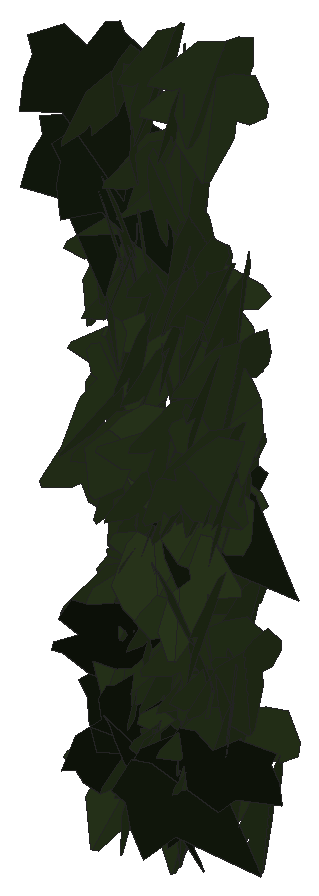
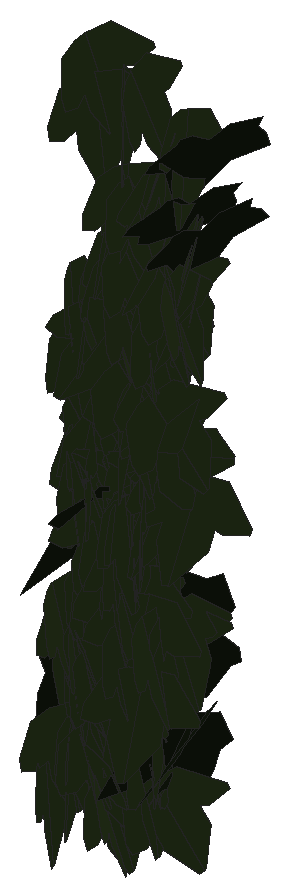
# SketchUp Ruby script. Lengths in inches.
U = 1.inch
M = Sketchup.active_model
def pt(a) = Geom::Point3d.new(a.map { |v| v * U })
def face(e, loops, mat)
  f = e.add_face(loops[0].map { |a| pt(a) })
  loops[1..].each { |l| e.add_face(l.map { |a| pt(a) }).erase! }
  f.material = f.back_material = mat if mat
  f
end
# faces: each face lists its corners as indices into pts; further lists are holes
def faces(e, pts, list, mat = nil) = list.each { |f| face(e, (f[0].is_a?(Array) ? f : [f]).map { |l| l.map { |i| pts[i] } }, mat) }
# xy, xz, yz: faces in a plane at the given z, y or x. An outline is a flat list of corners, or four numbers for a rectangle; further outlines are holes
def ring(l) = l.size == 4 ? [[l[0], l[1]], [l[2], l[1]], [l[2], l[3]], [l[0], l[3]]] : l.each_slice(2).to_a
def flat(e, list, mat, &to3) = list.each { |f| face(e, (f[0].is_a?(Array) ? f : [f]).map { |l| ring(l).map { |u, v| to3.(u, v) } }, mat) }
def xy(e, z, list, mat = nil) = flat(e, list, mat) { |x, y| [x, y, z] }
def xz(e, y, list, mat = nil) = flat(e, list, mat) { |x, z| [x, y, z] }
def yz(e, x, list, mat = nil) = flat(e, list, mat) { |y, z| [x, y, z] }
def lines(e, pts, list) = list.each { |a, b| e.add_line(pt(pts[a]), pt(pts[b])) }
# prism: a flat outline (further loops are holes) pulled along v
def prism(e, loops, v, mat = nil)
  f = face(e, loops, mat); d = Geom::Vector3d.new(v.map { |x| x * U })
  f.pushpull(f.normal.samedirection?(d) ? d.length : -d.length)
end
def box(e, o, s, mat = nil) = prism(e, [[o, [o[0] + s[0], o[1], o[2]], [o[0] + s[0], o[1] + s[1], o[2]], [o[0], o[1] + s[1], o[2]]]], [0, 0, s[2]], mat)
def at(x, y, z, deg = 0) = Geom::Transformation.translation(pt([x, y, z])) * Geom::Transformation.rotation(ORIGIN, Z_AXIS, deg.degrees)
def axes(o, x, y, z) = Geom::Transformation.new([*x, 0, *y, 0, *z, 0, *pt(o).to_a, 1])
def part(name) = M.definitions.add(name)
# library, detail: a bought-in or finely detailed component or shape, given as its bounding box
def library(name, o, s) = part(name).tap { |d| box(d.entities, o, s) }
def detail(e, o, s) = box(e.add_group.entities, o, s)
def put(e, d, t, mat = nil) = e.add_instance(d, t).tap { |i| i.material = mat if mat }
def group(e, t, mat = nil) = e.add_group.tap { |g| g.transformation = t; g.material = mat if mat }.entities
root = M.entities
M.materials.add("efeu1").color = [18, 25, 13]
M.materials.add("efeu2").color = [43, 57, 29]
c1 = part("ivyleaf_10")
p = [[0,0.5,-0.03],[-0.0625,2.02,-0.43],[-0.19,2.01,-0.46],[-0.54,1.05,-0.29],[-0.52,0.625,-0.18],[-0.83,0.76,-0.28],
  [-1.16,0.64,-0.33],[-1.15,0.33,-0.24],[-0.77,-0.39,0.02],[-0.3,-0.51,0.16],[0.04,-0.48,0.23],[-0.02,2.01,-0.4375],
  [-0.06,2.01,-0.43],[0.04,-0.49,0.23],[0.67,-0.49,0.14],[1.38,0.36,-0.2],[1.375,0.51,-0.24],[0.81,0.65,-0.19],
  [0.62,0.59,-0.15],[0.6,1.09,-0.28],[0.5,1.23,-0.31]]
faces(c1.entities,p,[[0,1,2,3,4,5,6,7,8,9,10],[11,12,0,13,14,15,16,17,18,19,20]],"efeu2")
c2 = part("ivyleaf_9")
p = [[1.54,2.16,1.25],[1.36,2.04,1.19],[-0.21,0.99,0.68],[-0.71,1.11,0.82],[-0.85,0.86,0.67],[-0.8,0.17,0.21],
  [-0.9,-0.01,0.1],[-0.67,-0.16,-0.02],[-0.08,-0.08,-0.05],[-0.03,-0.6,-0.4],[0.65,-0.88,-0.66],[0.83,-0.6,-0.49],
  [1.29,-0.42,-0.43],[1.8125,-0.07,-0.26],[1.21,0.44,0.15]]
faces(c2.entities,p,[[0,1,2,3,4,5,6,7,8,9,10,11,12,13,14]],"efeu1")
put(root,c1,axes([17.82,224.84,220.2],[-0.19535,0.15051,0.43495],[-0.41062,0.15646,-0.23857],[-0.20792,-0.45041,0.06247]))
put(root,c1,axes([17.64,225.125,214.26],[-0.27754,-0.33916,0.24072],[-0.06692,-0.2492,-0.42827],[0.41048,-0.26994,0.09294]))
put(root,c1,axes([17.58,225.38,216.36],[0.07877,-0.49372,0.0058],[-0.01202,-0.00779,-0.49979],[0.49361,0.0786,-0.0131]))
put(root,c1,axes([17.58,224.9375,216.29],[-0.0576,-0.48543,0.10507],[0.02083,-0.10805,-0.48774],[0.49623,-0.05181,0.03267]))
put(root,c1,axes([17.58,224.95,220.32],[0.14734,-0.47167,0.0763],[0.00938,-0.07698,-0.49395],[0.4777,0.14699,-0.01384]))
put(root,c1,axes([17.54,225,218.48],[0.02516,-0.19881,0.45809],[0.0849,-0.45029,-0.20008],[0.4921,0.08786,0.0111]))
put(root,c1,axes([17.56,224.68,217.81],[-0.3643,-0.31873,-0.12527],[0.106,0.06897,-0.48374],[0.32565,-0.37902,0.01731]))
put(root,c2,axes([17.43,224.68,221.13],[-0.03274,-0.49,-0.09395],[0.01592,0.09308,-0.491],[0.49867,-0.03515,0.00951]))
put(root,c1,axes([17.72,225.02,218.9],[-0.17217,-0.40927,0.2299],[-0.09402,-0.20985,-0.44399],[0.45991,-0.19611,-0.0047]))
put(root,c2,axes([17.42,224.59,222.19],[-0.0177,-0.45685,-0.20243],[0.04052,0.20057,-0.45621],[0.49804,-0.03255,0.02992]))
put(root,c1,axes([17.65,225.5,215.74],[-0.40878,-0.28117,-0.06194],[0.0531,0.0321,-0.49614],[0.28298,-0.4122,0.00362]))
put(root,c1,axes([17.67,225.2,215.36],[0.21033,-0.41833,-0.17538],[-0.01592,0.1864,-0.46368],[0.45333,0.20064,0.06509]))
put(root,c2,axes([17.43,225.04,214.93],[0.27553,-0.41045,-0.07496],[-0.02858,0.07105,-0.4941],[0.41625,0.27656,0.01569]))
put(root,c1,axes([17.79,224.88,216.14],[-0.26923,-0.38423,0.17287],[0.00236,-0.20652,-0.45535],[0.42132,-0.24438,0.11302]))
put(root,c2,axes([17.71,224.51,214.99],[-0.01891,0.09801,-0.48993],[-0.15122,0.46617,0.0991],[0.47621,0.15192,0.01201]))
put(root,c1,axes([17.6875,224.625,220.01],[-0.11774,0.4595,-0.15811],[0.04187,-0.15249,-0.47434],[-0.48413,-0.12494,-0.00257]))
put(root,c1,axes([17.84,225.05,214.6],[0.00748,-0.49315,-0.08217],[-0.01236,0.08197,-0.49308],[0.49979,0.0094,-0.01096]))
put(root,c1,axes([17.8,225.26,216.5],[-0.44354,-0.22205,-0.06299],[0.06918,0.00229,-0.49519],[0.2202,-0.44798,0.02869]))
put(root,c1,axes([17.81,224.38,220.77],[-0.31173,0.38758,0.05108],[-0.03602,0.03658,-0.49736],[-0.38927,-0.31376,0.00511]))
put(root,c1,axes([17.84,224.4,222.0625],[-0.02605,-0.46702,-0.17668],[0.01458,0.17614,-0.46772],[0.49911,-0.02952,0.00444]))
put(root,c1,axes([17.89,224.68,220.3125],[-0.11306,-0.43868,0.21161],[-0.02821,-0.21098,-0.45243],[0.48623,-0.11424,0.02296]))
put(root,c1,axes([17.86,224.42,220.83],[-0.34948,0.35429,0.04837],[-0.03125,0.03712,-0.49764],[-0.35621,-0.35085,-0.0038]))
put(root,c1,axes([17.9,224.69,218.1875],[-0.06353,-0.48532,0.10213],[0.01206,-0.10444,-0.48882],[0.4958,-0.05965,0.02497]))
put(root,c1,axes([17.9375,224.8,219.75],[-0.05129,-0.49183,0.07401],[-0.00551,-0.07383,-0.49449],[0.49733,-0.05154,0.00216]))
put(root,c1,axes([17.92,225.42,216.17],[0.0371,-0.49856,-0.00771],[-0.00015,0.00772,-0.49994],[0.49862,0.0371,0.00042]))
put(root,c1,axes([17.9,224.74,217.83],[-0.08485,-0.39683,-0.2921],[0.08334,0.28057,-0.40538],[0.48565,-0.11748,0.01853]))
put(root,c1,axes([18.07,225.07,218.89],[-0.17185,0.33504,0.32896],[-0.2317,0.24417,-0.36973],[-0.40839,-0.27951,0.07133]))
put(root,c1,axes([18.07,224.42,220.39],[0.13783,-0.35073,-0.32863],[-0.13362,0.30043,-0.37668],[0.46168,0.19165,-0.01091]))
put(root,c2,axes([17.73,224.5625,221.28],[0.08031,-0.42076,-0.25789],[0.03463,0.26544,-0.4223],[0.49229,0.04997,0.07178]))
put(root,c2,axes([17.61,224.31,215.98],[0.38879,0.10879,0.29497],[0.28815,0.06431,-0.40352],[-0.12574,0.48377,-0.01269]))
put(root,c1,axes([17.99,225.07,216.55],[0.05599,-0.48301,0.11648],[0.01291,-0.11577,-0.48624],[0.49669,0.05746,-0.00049]))
put(root,c1,axes([18,224.98,217.81],[0.23182,-0.37514,-0.23564],[-0.03826,0.24801,-0.43247],[0.44136,0.21854,0.08628]))
put(root,c1,axes([18.04,225.19,216.76],[-0.42345,-0.26588,-0.00128],[-0.00235,0.00615,-0.49996],[0.26587,-0.4234,-0.00646]))
put(root,c1,axes([18.09,224.44,221.76],[0.12173,-0.0932,-0.47591],[-0.08733,0.47844,-0.11604],[0.47703,0.11138,0.10021]))
put(root,c1,axes([18.06,225.16,217.56],[-0.07619,-0.4931,-0.03234],[0.00838,0.03143,-0.49894],[0.49409,-0.07657,0.00348]))
put(root,c1,axes([17.99,224.75,214.61],[0.20222,-0.44099,0.12096],[0.068,-0.10179,-0.48478],[0.4522,0.21252,0.0188]))
put(root,c1,axes([18.0625,225.02,218.9],[0.06683,-0.49525,-0.01612],[-0.00695,0.01533,-0.49972],[0.49547,0.06701,-0.00484]))
put(root,c1,axes([18.04,225.04,216.83],[-0.0728,-0.37306,0.32485],[0.06756,-0.33277,-0.36701],[0.49004,-0.00954,0.09886]))
put(root,c1,axes([18.08,224.625,219.35],[0.17556,-0.45547,-0.10828],[-0.01729,0.10926,-0.48761],[0.46785,0.17495,0.02261]))
put(root,c1,axes([18.01,224.8125,220.55],[-0.17848,0.46668,0.01896],[-0.01266,0.01545,-0.4996],[-0.46689,-0.17882,0.0063]))
put(root,c1,axes([18.19,225,219.15],[-0.25319,-0.35221,0.24869],[-0.06265,-0.25528,-0.42533],[0.42658,-0.24654,0.08514]))
put(root,c1,axes([18.14,225.18,216.99],[0.05901,-0.48372,-0.11196],[-0.01565,0.11088,-0.4873],[0.49626,0.06102,-0.00205]))
put(root,c2,axes([17.77,224.84,214.6],[0.32355,-0.35467,0.13974],[0.09122,-0.10592,-0.48006],[0.37013,0.33614,-0.00383]))
put(root,c1,axes([18.4,224.72,215.84],[-0.35572,-0.04393,0.34862],[-0.33969,-0.08386,-0.35718],[0.08985,-0.49096,0.02982]))
put(root,c1,axes([18.1875,224.85,217.5625],[0.15468,-0.40897,-0.24253],[-0.05545,0.23778,-0.43633],[0.47223,0.16188,0.0282]))
put(root,c1,axes([18.16,224.92,216.3],[0.10616,-0.48859,-0.00244],[0.00163,0.00285,-0.49999],[0.4886,0.10615,0.0022]))
put(root,c1,axes([18.15,225.1,217.5],[0.06009,-0.48239,-0.117],[0.04698,0.12286,-0.48239],[0.49415,0.04698,0.06009]))
put(root,c1,axes([18.2,224.96,220.65],[-0.06784,-0.4687,0.16036],[0.00635,-0.16267,-0.47276],[0.49534,-0.0621,0.02802]))
put(root,c1,axes([18.19,224.98,214.83],[-0.01164,-0.49155,-0.09078],[0.00961,0.09057,-0.49163],[0.49977,-0.01319,0.00734]))
put(root,c1,axes([18.22,224.94,217.51],[-0.03507,-0.49843,0.01845],[-0.00112,-0.01842,-0.49966],[0.49877,-0.03509,0.00017]))
put(root,c1,axes([18.1875,224.8,217.05],[0.09673,-0.4734,0.1286],[0.02845,-0.12544,-0.48317],[0.48973,0.10079,0.00267]))
put(root,c1,axes([18.26,224.77,221.27],[-0.09398,-0.48567,0.07272],[-0.02848,-0.06852,-0.49446],[0.49026,-0.09709,-0.01478]))
put(root,c1,axes([18.3,225.4,214.84],[-0.29807,-0.36187,0.17379],[-0.06066,-0.17338,-0.46504],[0.39683,-0.29832,0.05946]))
put(root,c1,axes([18.23,224.99,220.05],[0.03325,-0.49322,0.07505],[-0.00643,-0.07563,-0.4942],[0.49885,0.0319,-0.01137]))
put(root,c1,axes([18.21,225.26,214.21],[-0.06442,-0.47993,0.12458],[0.04317,-0.13058,-0.48071],[0.49395,-0.05118,0.05826]))
put(root,c1,axes([18.26,225.15,217.11],[-0.13533,0.46818,0.11175],[-0.14192,0.07211,-0.47398],[-0.45994,-0.16001,0.11337]))
put(root,c1,axes([18.1,224.75,217.42],[-0.35048,-0.2125,-0.28637],[0.26167,0.11952,-0.40895],[0.24226,-0.43653,0.02743]))
put(root,c1,axes([18.17,225.02,214.62],[-0.47717,-0.00799,-0.14914],[0.14895,0.0111,-0.47717],[0.01094,-0.49981,-0.00822]))
put(root,c1,axes([18.28,225.27,214.24],[0.17444,-0.46814,0.02036],[0.00766,-0.01887,-0.49959],[0.46852,0.17461,0.00059]))
put(root,c1,axes([18.08,224.39,218.23],[-0.2791,-0.23811,-0.33971],[0.30948,0.15316,-0.36162],[0.27627,-0.41212,0.06188]))
put(root,c1,axes([18.35,224.55,221.18],[-0.18082,0.40361,0.23324],[-0.12576,0.19866,-0.44127],[-0.44888,-0.21824,0.02968]))
put(root,c1,axes([18.33,224.91,215.79],[0.05316,-0.48049,-0.1277],[0.00479,0.12891,-0.48307],[0.49714,0.05014,0.01831]))
put(root,c1,axes([18.34,224.83,221.4],[-0.21261,-0.45051,-0.04288],[0.05107,0.02319,-0.49684],[0.44965,-0.21565,0.03616]))
put(root,c1,axes([18.32,224.62,222.52],[0.09329,-0.46685,0.15279],[0.04881,-0.14595,-0.47573],[0.48879,0.10368,0.01834]))
put(root,c1,axes([18.42,225.03,216.56],[-0.24638,-0.41095,0.14289],[-0.03399,-0.14553,-0.47714],[0.43375,-0.24483,0.04377]))
put(root,c1,axes([18.38,225.35,215.7],[-0.02165,-0.48305,0.12725],[0.02552,-0.12827,-0.48259],[0.49888,-0.0144,0.03021]))
put(root,c1,axes([18.52,224.5,218.16],[-0.37278,-0.28771,0.1681],[-0.13398,-0.10152,-0.47089],[0.30509,-0.39613,-0.00141]))
put(root,c1,axes([18.41,224.5625,217.88],[-0.11289,-0.48482,-0.04698],[0.00612,0.04681,-0.49777],[0.48705,-0.11296,-0.00463]))
put(root,c1,axes([18.44,224.47,216.79],[-0.38729,0.28905,0.12829],[-0.09293,0.08986,-0.483],[-0.30228,-0.39796,-0.01588]))
put(root,c1,axes([18.34,225.13,217.41],[-0.39275,-0.27471,-0.14243],[0.16335,0.01141,-0.47243],[0.26281,-0.41762,0.08079]))
put(root,c1,axes([18.51,225.35,215.95],[0.39243,-0.18867,-0.24577],[-0.17127,0.19842,-0.42579],[0.2582,0.41837,0.09111]))
put(root,c1,axes([18.42,225,217.2],[-0.08522,-0.49151,0.03393],[0.04824,-0.0426,-0.49584],[0.49032,-0.08123,0.05468]))
put(root,c1,axes([18.41,224.83,219.7],[0.25346,-0.42883,0.04323],[0.01745,-0.0399,-0.4981],[0.43065,0.254,-0.00526]))
put(root,c1,axes([18.47,225.2,215.53],[-0.01022,-0.49973,0.01279],[-0.00403,-0.01271,-0.49982],[0.49988,-0.01032,-0.00377]))
put(root,c1,axes([18.32,225.48,214.7],[0.44477,-0.19646,0.11655],[0.10263,-0.05604,-0.48613],[0.20407,0.45636,-0.00952]))
put(root,c1,axes([18.4375,225.17,214.46],[0.18628,-0.45257,0.10238],[0.03159,-0.0977,-0.48934],[0.46293,0.18878,-0.00781]))
put(root,c1,axes([18.78,224.54,215.84],[-0.05206,0.07251,-0.49197],[-0.39015,0.30076,0.08562],[0.30834,0.3928,0.02526]))
put(root,c1,axes([18.82,224.62,215.9],[-0.2264,0.0186,0.44542],[-0.44378,0.03813,-0.22716],[-0.04242,-0.4982,-0.00076]))
put(root,c1,axes([18.38,224.61,217.68],[0.22106,0.21501,-0.39358],[0.2232,0.32785,0.30446],[0.38899,-0.3103,0.04896]))
put(root,c1,axes([18.6,225.36,215.87],[0.16209,-0.44913,-0.14836],[-0.03339,0.14557,-0.47717],[0.47182,0.1646,0.01719]))
put(root,c1,axes([18.6,224.6,218.62],[0.00605,-0.49288,0.08383],[-0.00441,-0.08389,-0.49289],[0.49994,0.00523,-0.00536]))
put(root,c1,axes([18.61,225.08,216],[-0.0918,-0.46829,0.14925],[0.00086,-0.15198,-0.47634],[0.4915,-0.0872,0.02871]))
put(root,c1,axes([18.42,224.29,216.68],[0.16282,0.23908,-0.40784],[0.24456,0.32655,0.28906],[0.40458,-0.29361,-0.0106]))
put(root,c1,axes([18.46,225,219.72],[-0.40149,-0.16987,-0.24485],[0.24226,0.05318,-0.43414],[0.17353,-0.46724,0.03961]))
put(root,c1,axes([18.67,224.96,216.57],[-0.10246,-0.47013,0.13595],[-0.02407,-0.13389,-0.48114],[0.4888,-0.10513,0.00481]))
put(root,c1,axes([18.62,224.7,217.89],[-0.02036,-0.42786,-0.25791],[0.03543,0.25624,-0.42789],[0.49833,-0.0357,0.01989]))
put(root,c1,axes([18.68,224.41,222.3],[0.1639,-0.38547,-0.27304],[-0.05583,0.27118,-0.41635],[0.46906,0.16697,0.04585]))
put(root,c1,axes([18.66,225.22,214.73],[-0.0216,-0.49945,-0.00889],[-0.00509,0.00911,-0.49989],[0.49951,-0.0215,-0.00548]))
put(root,c1,axes([18.69,225.07,218.22],[0.24728,-0.30878,-0.30579],[-0.09589,0.30438,-0.38491],[0.42386,0.24901,0.09132]))
put(root,c1,axes([18.7,224.39,220.39],[0.2562,-0.40076,-0.15412],[-0.06838,0.1391,-0.47537],[0.42389,0.26466,0.01647]))
put(root,c1,axes([18.66,225.01,214.78],[0.1117,-0.48168,0.0742],[0.01439,-0.07284,-0.49446],[0.48715,0.1126,-0.00241]))
put(root,c1,axes([18.57,225.34,215.99],[0.33533,-0.35351,0.11219],[0.07819,-0.08047,-0.48725],[0.36255,0.34432,0.00131]))
put(root,c1,axes([18.6875,225,217.92],[-0.11378,-0.48499,-0.04284],[0.01286,0.04098,-0.49815],[0.48671,-0.11446,0.00315]))
put(root,c1,axes([18.77,224.76,217.62],[-0.3146,-0.29829,0.24909],[-0.05691,-0.28167,-0.40918],[0.38443,-0.28581,0.14328]))
put(root,c1,axes([18.66,225.1,218.5625],[0.06984,0.35008,-0.35009],[-0.06793,-0.34344,-0.35698],[-0.49042,0.09742,-0.00041]))
put(root,c1,axes([18.73,225.375,214.88],[-0.31022,-0.38553,0.07162],[0.02227,-0.10849,-0.48758],[0.39149,-0.29933,0.08448]))
put(root,c1,axes([18.58,224.52,217.07],[0.48145,0.12865,0.04067],[0.03771,0.01638,-0.49831],[-0.12955,0.48289,0.00607]))
put(root,c1,axes([18.73,225.24,214.59],[0.156,-0.41879,-0.22422],[0.00255,0.23674,-0.4404],[0.47503,0.13626,0.076]))
put(root,c2,axes([18.51,224.96,217.53],[0.16313,-0.28573,-0.37649],[-0.04735,0.3864,-0.31377],[0.47026,0.13803,0.09901]))
put(root,c1,axes([18.78,225.43,216.38],[0.10177,-0.48941,-0.01114],[-0.00535,0.01027,-0.49987],[0.48951,0.10186,-0.00314]))
put(root,c1,axes([18.78,224.45,220.85],[0.08982,-0.36434,-0.33044],[0.00122,0.33607,-0.37021],[0.49186,0.0657,0.06126]))
put(root,c1,axes([18.66,224.84,218.2],[0.04035,-0.25749,0.4267],[0.16695,-0.39638,-0.25497],[0.46957,0.16305,0.05399]))
put(root,c1,axes([18.8,224.74,216.13],[-0.30194,-0.39322,-0.06493],[0.03171,0.0575,-0.49567],[0.39728,-0.30344,-0.00979]))
put(root,c2,axes([18.55,224.33,214.83],[0.20575,-0.30246,-0.34086],[-0.04881,0.35721,-0.34643],[0.45308,0.17583,0.11747]))
put(root,c1,axes([18.77,224.75,220.04],[0.0952,-0.43055,-0.23572],[0.06534,0.24909,-0.42858],[0.48648,0.0508,0.1037]))
put(root,c1,axes([18.8125,224.78,219.98],[0.10926,-0.46651,0.14292],[0.0269,-0.14048,-0.47911],[0.48717,0.11238,-0.00559]))
put(root,c1,axes([18.86,224.92,218.01],[-0.07423,-0.4541,-0.19567],[0.01936,0.19504,-0.45998],[0.49408,-0.07587,-0.01138]))
put(root,c1,axes([18.85,224.8125,215.71],[0.07138,-0.44941,0.2072],[0.02304,-0.2061,-0.45496],[0.49434,0.0745,-0.00871]))
put(root,c1,axes([18.88,224.77,215.24],[-0.05192,-0.48634,0.10379],[0.00425,-0.10479,-0.48888],[0.49728,-0.04988,0.01502]))
put(root,c1,axes([18.85,224.42,220.28],[-0.02376,-0.45906,-0.19673],[0.04935,0.19383,-0.45825],[0.49699,-0.04119,0.0361]))
put(root,c1,axes([18.91,224.98,218.07],[0.13378,-0.44737,-0.17878],[-0.03411,0.17629,-0.46665],[0.48056,0.13705,0.01665]))
put(root,c1,axes([18.87,224.67,219.15],[0.24658,-0.43078,0.06023],[0.01885,-0.05858,-0.4962],[0.43456,0.24697,-0.01265]))
put(root,c1,axes([18.94,224.625,222.23],[-0.30404,-0.39381,0.04974],[0.00233,-0.06443,-0.49583],[0.39693,-0.30127,0.04101]))
put(root,c2,axes([19.03,224.48,215.1],[0.18807,0.2964,-0.35606],[-0.18371,-0.30507,-0.35098],[-0.4253,0.26284,-0.00584]))
put(root,c1,axes([18.8125,225.11,217.97],[0.38985,-0.29171,0.11369],[0.08599,-0.07482,-0.48683],[0.30104,0.39914,-0.00817]))
put(root,c1,axes([19.125,224.85,218.76],[0.3004,-0.2254,-0.33008],[-0.2699,0.19016,-0.37549],[0.29481,0.40378,-0.00742]))
put(root,c1,axes([18.95,225.4,214.24],[0.11584,-0.47898,-0.08464],[0.02182,0.09203,-0.49097],[0.48591,0.11006,0.04222]))
put(root,c1,axes([19.02,224.56,222.68],[-0.125,-0.47006,0.11584],[-0.01991,-0.11454,-0.4863],[0.48371,-0.12619,0.00992]))
put(root,c1,axes([19.03,224.83,219.28],[-0.0852,-0.49228,0.01992],[-0.00333,-0.01964,-0.4996],[0.49268,-0.08527,0.00007]))
put(root,c1,axes([18.96,224.6,216.79],[0.24798,-0.4219,0.10251],[0.03796,-0.09653,-0.48912],[0.43251,0.25037,-0.01584]))
put(root,c1,axes([19.06,224.59,218.43],[-0.01922,-0.48427,0.12295],[-0.01968,-0.12221,-0.48444],[0.49924,-0.02346,-0.01437]))
put(root,c1,axes([19.01,224.89,219.98],[0.14931,-0.46699,-0.09811],[0.0152,0.10741,-0.48809],[0.47694,0.14277,0.04628]))
put(root,c1,axes([19.01,224.82,218],[0.26447,-0.42328,0.02981],[0.01145,-0.02799,-0.49908],[0.42417,0.26467,-0.00511]))
put(root,c1,axes([19.05,224.71,215.76],[0.32452,-0.35389,-0.13947],[-0.02398,0.16393,-0.47175],[0.37962,0.31287,0.08943]))
put(root,c1,axes([19.07,224.89,215.91],[-0.07862,-0.47581,-0.13199],[0.02193,0.13016,-0.48226],[0.49329,-0.08163,0.0004]))
put(root,c1,axes([19,224.26,218.27],[-0.23738,-0.35348,-0.26212],[0.13217,0.2268,-0.42555],[0.41974,-0.27132,-0.01424]))
